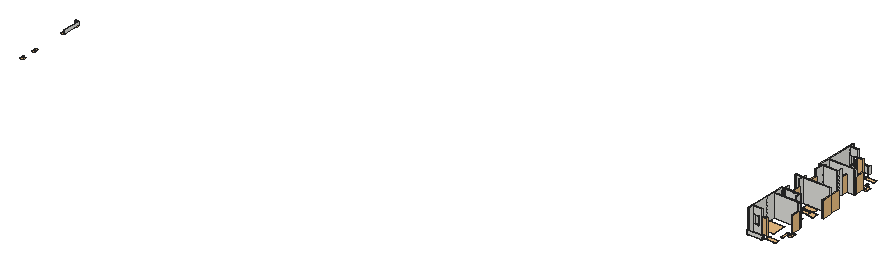
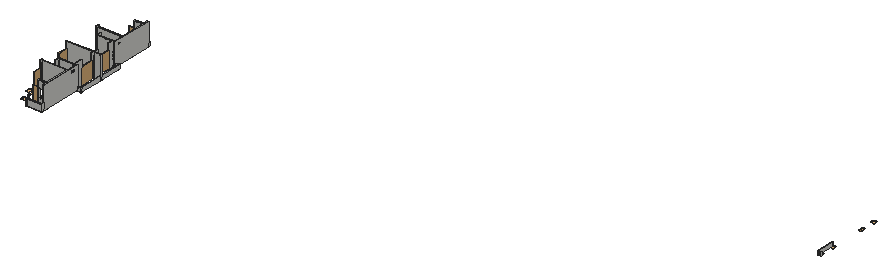
# SketchUp Ruby script. Lengths in inches.
U = 1.inch
M = Sketchup.active_model
def pt(a) = Geom::Point3d.new(a.map { |v| v * U })
def face(e, loops, mat)
  f = e.add_face(loops[0].map { |a| pt(a) })
  loops[1..].each { |l| e.add_face(l.map { |a| pt(a) }).erase! }
  f.material = f.back_material = mat if mat
  f
end
# faces: each face lists its corners as indices into pts; further lists are holes
def faces(e, pts, list, mat = nil) = list.each { |f| face(e, (f[0].is_a?(Array) ? f : [f]).map { |l| l.map { |i| pts[i] } }, mat) }
# xy, xz, yz: faces in a plane at the given z, y or x. An outline is a flat list of corners, or four numbers for a rectangle; further outlines are holes
def ring(l) = l.size == 4 ? [[l[0], l[1]], [l[2], l[1]], [l[2], l[3]], [l[0], l[3]]] : l.each_slice(2).to_a
def flat(e, list, mat, &to3) = list.each { |f| face(e, (f[0].is_a?(Array) ? f : [f]).map { |l| ring(l).map { |u, v| to3.(u, v) } }, mat) }
def xy(e, z, list, mat = nil) = flat(e, list, mat) { |x, y| [x, y, z] }
def xz(e, y, list, mat = nil) = flat(e, list, mat) { |x, z| [x, y, z] }
def yz(e, x, list, mat = nil) = flat(e, list, mat) { |y, z| [x, y, z] }
def lines(e, pts, list) = list.each { |a, b| e.add_line(pt(pts[a]), pt(pts[b])) }
# prism: a flat outline (further loops are holes) pulled along v
def prism(e, loops, v, mat = nil)
  f = face(e, loops, mat); d = Geom::Vector3d.new(v.map { |x| x * U })
  f.pushpull(f.normal.samedirection?(d) ? d.length : -d.length)
end
def box(e, o, s, mat = nil) = prism(e, [[o, [o[0] + s[0], o[1], o[2]], [o[0] + s[0], o[1] + s[1], o[2]], [o[0], o[1] + s[1], o[2]]]], [0, 0, s[2]], mat)
def at(x, y, z, deg = 0) = Geom::Transformation.translation(pt([x, y, z])) * Geom::Transformation.rotation(ORIGIN, Z_AXIS, deg.degrees)
def axes(o, x, y, z) = Geom::Transformation.new([*x, 0, *y, 0, *z, 0, *pt(o).to_a, 1])
def part(name) = M.definitions.add(name)
# library, detail: a bought-in or finely detailed component or shape, given as its bounding box
def library(name, o, s) = part(name).tap { |d| box(d.entities, o, s) }
def detail(e, o, s) = box(e.add_group.entities, o, s)
def put(e, d, t, mat = nil) = e.add_instance(d, t).tap { |i| i.material = mat if mat }
def group(e, t, mat = nil) = e.add_group.tap { |g| g.transformation = t; g.material = mat if mat }.entities
root = M.entities
M.materials.add("M09_Shadow_Night").color = [0, 0, 0]
c1 = library("TREE-26",[-60.96,-72.91,0],[121.92,134.74,0.01])
c2 = part("Group\#14")
xy(c2.entities,0,[[0,0,4.05,3.45],[0,3.45,4.05,88.84],[-13.95,88.84,0,93],[0,88.84,4.05,93]])
xy(c2.entities,18,[[0,0,4.05,88.84],[-13.95,88.84,0,93],[0,88.84,4.05,93]],"M09_Shadow_Night")
xz(c2.entities,0,[[0,0,4.05,18]])
xz(c2.entities,88.84,[[-13.95,0,0,18]])
xz(c2.entities,93,[[-13.95,0,4.05,18]])
yz(c2.entities,-13.95,[[88.84,0,93,18]])
yz(c2.entities,0,[[0,0,3.45,18],[3.45,0,88.84,18]])
yz(c2.entities,4.05,[[0,0,93,18]])
c3 = library("porta correr aluminio",[0,0,0],[4.49,110.28,83.35])
c4 = library("ghgjg",[-265.23,-341.01,0],[530.46,682.02,0.01])
c5 = library("VVVV",[-3.39,-3.68,0],[6.78,7.36,0.01])
c6 = part("Group\#13")
xy(c6.entities,0,[[0,0,4,3.01],[80,0,84,8],[0,3.01,4,8],[0,8,4,12],[4,8,80,12],
  [80,8,84,12]])
xy(c6.entities,36,[[0,0,4,12],[80,0,84,12],[4,8,80,12]],"M09_Shadow_Night")
xz(c6.entities,0,[[0,0,4,36],[80,0,84,36]])
xz(c6.entities,8,[[4,0,80,36]])
xz(c6.entities,12,[[0,0,80,36],[80,0,84,36]])
yz(c6.entities,0,[[0,0,12,36]])
yz(c6.entities,4,[[0,0,3.01,36],[3.01,0,8,36]])
yz(c6.entities,80,[[0,0,8,36],[8,0,12,36]])
yz(c6.entities,84,[[0,0,12,36]])
c7 = part("Group\#6")
xy(c7.entities,0,[[0,-8,80,-4],[80,-8,84,-4],[0,-4,4,0],[80,-4,84,4],[0,0,4,4]])
xy(c7.entities,20,[[0,-8,84,-8,84,4,80,4,80,-4,4,-4,4,4,0,4]],"M09_Shadow_Night")
xz(c7.entities,-8,[[0,0,84,20]])
xz(c7.entities,-4,[[4,0,80,20]])
xz(c7.entities,4,[[0,0,4,20],[80,0,84,20]])
yz(c7.entities,0,[[-8,0,4,20]])
yz(c7.entities,4,[[-4,0,0,20],[0,0,4,20]])
yz(c7.entities,80,[[-4,0,4,20]])
yz(c7.entities,84,[[-8,0,-4,20],[-4,0,4,20]])
c8 = library("double bed",[-999.9375,-1062.5,0],[1999.875,2125,0.01])
c9 = part("tgr")
p = [[-2.37,-3.35,0],[-2.37,-2.82,0],[-2.73,-2.82,0],[-2.73,-2.68,0],[-3.71,-2.68,0],[-3.71,-3.35,0],
  [-2.37,3.35,0],[-2.37,2.82,0],[-2.73,2.82,0],[-2.73,2.68,0],[-3.71,2.68,0],[-3.71,3.35,0],
  [3.71,-2.82,0],[-2.37,-2.46,0],[3.71,-2.46,0],[3.7,-2.46,0],[3.63,-2.07,0],[3.53,-1.68,0],
  [3.41,-1.3,0],[3.27,-0.93,0],[3.1,-0.57,0],[2.91,-0.22,0],[2.7,0.12,0],[2.46,0.4375,0],
  [2.21,0.74,0],[1.93,1.03,0],[1.64,1.3,0],[1.33,1.55,0],[1.01,1.79,0],[0.67,1.99,0],
  [0.32,2.18,0],[-0.04,2.35,0],[-0.41,2.49,0],[-0.8,2.6,0],[-1.18,2.69,0],[-1.58,2.76,0],
  [-1.97,2.8,0]]
lines(c9.entities,p,[[0,1],[1,2],[2,3],[3,4],[4,5],[5,0],[6,7],[7,8],[8,9],[9,10],[10,11],[11,6],
  [1,12],[13,14],[1,13],[12,14],[15,16],[16,17],[17,18],[18,19],[19,20],[20,21],[21,22],[22,23],
  [23,24],[24,25],[25,26],[26,27],[27,28],[28,29],[29,30],[30,31],[31,32],[32,33],[33,34],[34,35],
  [35,36],[36,7]])
c10 = library("Group\#51",[0,0,0],[6.9375,42,86.5])
c11 = library("HYHHYHYHYHYHY",[-2.09,-4.54,0],[4.18,9.08,0.01])
c12 = library("BFGFV",[-4.32,-2.51,0],[8.64,5.02,0.01])
c13 = library("lcd-01",[-577.99,-134.75,0],[1155.98,269.5,0.01])
c14 = library("JEEW",[-211.14,-299.86,0],[422.28,599.72,0.01])
c15 = library("Group\#49",[0,0,0],[8.31,30,84])
c16 = library("Component\#1",[961.32,38.58,0],[54,24,0.01])
c17 = library("Component\#3",[961.32,686.58,0],[54,18,0.01])
c18 = part("EGWF")
p = [[2.59,-3.49,0],[2.59,-3.09,0],[2.85,-3.09,0],[2.85,-2.99,0],[3.58,-2.99,0],[3.58,-3.49,0],
  [2.59,3.49,0],[2.59,3.09,0],[2.85,3.09,0],[2.85,2.99,0],[3.58,2.99,0],[3.58,3.49,0],
  [-3.58,-3.09,0],[2.59,-2.82,0],[-3.58,-2.82,0],[2.2,3.07,0],[1.81,3.04,0],[1.42,2.97,0],
  [1.03,2.89,0],[0.66,2.78,0],[0.29,2.64,0],[-0.07,2.48,0],[-0.42,2.3,0],[-0.76,2.1,0],
  [-1.08,1.875,0],[-1.39,1.63,0],[-1.68,1.37,0],[-1.96,1.09,0],[-2.21,0.79,0],[-2.45,0.48,0],
  [-2.67,0.15,0],[-2.86,-0.1875,0],[-3.04,-0.54,0],[-3.1875,-0.9,0],[-3.32,-1.28,0],[-3.42,-1.66,0],
  [-3.5,-2.04,0],[-3.55,-2.43,0]]
lines(c18.entities,p,[[0,1],[1,2],[2,3],[3,4],[4,5],[5,0],[6,7],[7,8],[8,9],[9,10],[10,11],[11,6],
  [1,12],[13,14],[1,13],[12,14],[7,15],[15,16],[16,17],[17,18],[18,19],[19,20],[20,21],[21,22],
  [22,23],[23,24],[24,25],[25,26],[26,27],[27,28],[28,29],[29,30],[30,31],[31,32],[32,33],[33,34],
  [34,35],[35,36],[36,37],[37,14]])
c19 = part("feeeeeeeeee")
p = [[-2.68,3.51,0],[-2.68,3.16,0],[-2.92,3.16,0],[-2.92,3.07,0],[-3.56,3.07,0],[-3.56,3.51,0],
  [-2.68,-3.51,0],[-2.68,-3.16,0],[-2.92,-3.16,0],[-2.92,-3.07,0],[-3.56,-3.07,0],[-3.56,-3.51,0],
  [3.56,3.16,0],[-2.68,2.93,0],[3.56,2.93,0],[-2.48,-3.13,0],[-2.04,-3.07,0],[-1.61,-2.98,0],
  [-1.1875,-2.86,0],[-0.77,-2.72,0],[-0.36,-2.55,0],[0.03,-2.35,0],[0.41,-2.13,0],[0.78,-1.88,0],
  [1.125,-1.62,0],[1.46,-1.32,0],[1.77,-1.01,0],[2.06,-0.68,0],[2.33,-0.33,0],[2.57,0.03,0],
  [2.79,0.42,0],[2.99,0.81,0],[3.16,1.22,0],[3.3,1.63,0],[3.41,2.06,0],[3.5,2.49,0]]
lines(c19.entities,p,[[0,1],[1,2],[2,3],[3,4],[4,5],[5,0],[6,7],[7,8],[8,9],[9,10],[10,11],[11,6],
  [1,12],[13,14],[1,13],[12,14],[8,15],[15,16],[16,17],[17,18],[18,19],[19,20],[20,21],[21,22],
  [22,23],[23,24],[24,25],[25,26],[26,27],[27,28],[28,29],[29,30],[30,31],[31,32],[32,33],[33,34],
  [34,35],[35,14]])
xy(root,246,[[3708.46,942.875,3762.46,966.875]])
put(root,c1,axes([371.8,298.64,246],[0,0.1317,0],[0.1317,0,0],[0,0,0.1317]))
put(root,c1,axes([371.8,222.26,246],[0,0.1317,0],[0.1317,0,0],[0,0,0.1317]))
put(root,c1,axes([371.8,567.61,246],[0,0.1317,0],[0.1317,0,0],[0,0,0.1317]))
put(root,c1,axes([371.8,491.09,246],[0,0.1317,0],[0.1317,0,0],[0,0,0.1317]))
put(root,c2,at(376.15,484.34,246))
put(root,c1,axes([3611.24,1266.81,246],[0,0.1317,0],[0.1317,0,0],[0,0,0.1317]))
put(root,c1,axes([3611.24,1401.53,246],[0,0.1317,0],[0.1317,0,0],[0,0,0.1317]))
put(root,c1,axes([3611.24,1285.67,246],[0,0.1317,0],[0.1317,0,0],[0,0,0.1317]))
put(root,c1,axes([3611.24,1162.38,246],[0,0.1317,0],[0.1317,0,0],[0,0,0.1317]))
put(root,c1,axes([3635.38,935.84,246],[0,0.1317,0],[0.1317,0,0],[0,0,0.1317]))
put(root,c1,axes([3637.36,1629.4,246],[0,0.1317,0],[0.1317,0,0],[0,0,0.1317]))
put(root,c3,axes([3644.59,1182.875,246.65],[-1.89519,0,0],[0,0.65291,0],[0,0,1]))
put(root,c3,axes([3644.59,1292.48,246.65],[-1.89519,0,0],[0,0.65291,0],[0,0,1]))
put(root,c4,axes([3644.1,1128.875,246],[0,-0.04,0],[-0.04,0,0],[0,0,0.04]))
put(root,c4,axes([3644.1,1434.875,246],[0,-0.04,0],[-0.04,0,0],[0,0,0.04]))
put(root,c5,axes([3663.08,1221.31,246],[4.47564,0,0],[0,-4.47564,0],[0,0,4.47564]))
put(root,c5,axes([3663.08,1330.86,246],[4.47564,0,0],[0,4.47564,0],[0,0,4.47564]))
put(root,c6,at(3624.46,1626.8,246))
put(root,c7,at(3624.46,932.875,246))
put(root,c8,axes([3669.72,1035.82,246],[0,-0.03695,0],[-0.03695,0,0],[0,0,0.03695]))
put(root,c8,axes([3669.72,1520.61,246],[0,-0.03695,0],[-0.03695,0,0],[0,0,0.03695]))
put(root,c9,axes([3687.46,1613.47,246],[0,4.47464,0],[-4.47464,0,0],[0,0,4.47464]))
put(root,c10,axes([3702.46,1595.22,246],[0,0.85622,0],[-0.71429,0,0],[0,0,0.97071]))
put(root,c9,axes([3687.46,950.27,246],[0,-4.47464,0],[-4.47464,0,0],[0,0,4.47464]))
put(root,c10,axes([3674.86,968.53,246],[0,-0.85622,0],[0.65714,0,0],[0,0,0.9711]))
g1 = group(root,at(3624.46,1619.08,246))
xy(g1,0,[[12,-255.51,18,-214.2],[0,-214.2,6,-208.2],[6,-214.2,12,-208.2],[12,-214.2,18,-208.2],[18,-214.2,94,-208.2],
  [94,-214.2,100,-208.2],[0,-208.2,6,-160.2],[94,-208.2,100,-190.2],[0,-160.2,6,-154.2],[6,-160.2,138,-154.2],
  [138,-160.2,144,-154.2],[0,-154.2,6,-116.77],[138,-154.2,144,-148.2],[0,-116.77,6,-80.17],[0,-80.17,6,-22.2],
  [0,-22.2,6,-16.2],[6,-22.2,48,-16.2],[0,-16.2,6,0],[0,0,6,7.73]])
xy(g1,36,[[8,-22.2,46,-16.2]])
xy(g1,84,[[8,-22.2,46,-16.2]])
xy(g1,96,[[0,-196.2,6,-172.2]])
xy(g1,108,[[0,-196.2,6,-172.2]])
xy(g1,120,[[12,-255.51,18,-214.2],[0,-214.2,6,-208.2],[6,-214.2,12,-208.2],[12,-214.2,18,-208.2],[18,-214.2,94,-208.2],
  [94,-214.2,100,-208.2],[0,-208.2,6,-160.2],[94,-208.2,100,-190.2],[0,-160.2,6,-154.2],[6,-160.2,138,-154.2],
  [138,-160.2,144,-154.2],[0,-154.2,6,-22.2],[138,-154.2,144,-148.2],[0,-22.2,6,-16.2],[6,-22.2,48,-16.2],
  [0,-16.2,6,0],[0,0,6,7.73]])
xz(g1,-255.51,[[12,0,18,120]])
xz(g1,-214.2,[[0,0,6,120],[6,0,12,120],[12,0,18,120],[18,0,94,120],[94,0,100,120]])
xz(g1,-208.2,[[6,0,12,120],[12,0,18,120],[18,0,94,120],[94,0,100,120]])
xz(g1,-196.2,[[0,96,6,108]])
xz(g1,-190.2,[[94,0,100,120]])
xz(g1,-172.2,[[0,96,6,108]])
xz(g1,-160.2,[[6,0,138,120],[138,0,144,120]])
xz(g1,-154.2,[[6,0,138,120],[138,0,144,120]])
xz(g1,-148.2,[[138,0,144,120]])
xz(g1,-22.2,[[[6,0,48,120],[8,36,46,84]]])
xz(g1,-16.2,[[[6,0,48,120],[8,36,46,84]]])
xz(g1,7.73,[[0,0,6,120]])
yz(g1,0,[[[-214.2,0,7.73,120],[-196.2,96,-172.2,108]]])
yz(g1,6,[[-214.2,0,-208.2,120],[[-208.2,0,-160.2,120],[-196.2,96,-172.2,108]],[-160.2,0,-154.2,120],[-154.2,0,-22.2,120],[-22.2,0,-16.2,120],
  [-16.2,0,0,120],[0,0,7.73,120]])
yz(g1,8,[[-22.2,36,-16.2,84]])
yz(g1,12,[[-255.51,0,-214.2,120],[-214.2,0,-208.2,120]])
yz(g1,18,[[-255.51,0,-214.2,120],[-214.2,0,-208.2,120]])
yz(g1,46,[[-22.2,36,-16.2,84]])
yz(g1,48,[[-22.2,0,-16.2,120]])
yz(g1,94,[[-214.2,0,-208.2,120],[-208.2,0,-190.2,120]])
yz(g1,100,[[-214.2,0,-208.2,120],[-208.2,0,-190.2,120]])
yz(g1,138,[[-160.2,0,-154.2,120],[-154.2,0,-148.2,120]])
yz(g1,144,[[-160.2,0,-154.2,120],[-154.2,0,-148.2,120]])
g2 = group(g1,at(-2.625,-212.2,0))
xy(g2,0,[[2.625,-470,8.625,-446],[2.625,-446,8.625,-440],[8.625,-446,53.03,-440],[2.625,-440,8.625,-352.75],[2.625,-352.75,8.625,-308],
  [140.625,-317.47,146.625,-308],[2.625,-308,8.625,-302],[8.625,-308,140.625,-302],[140.625,-308,146.625,-302],[2.625,-302,8.625,-254],
  [96.625,-272,102.625,-254],[-21.375,-254,-17.27,-250],[-17.27,-254,2.625,-250],[2.625,-254,8.625,-250],[8.625,-254,14.625,-250],
  [14.625,-254,20.625,-250],[20.625,-254,96.625,-250],[96.625,-254,102.625,-250],[-21.375,-250,-17.27,-133.43],[2.625,-250,8.625,-248],
  [8.625,-250,14.625,-248],[14.625,-250,20.625,-248],[20.625,-250,96.625,-248],[96.625,-250,102.625,-248],[14.625,-248,20.625,-224],
  [14.625,-152,20.625,-133.43],[-21.375,-133.43,-17.27,-127.79],[-17.27,-133.43,14.625,-127.79],[14.625,-133.43,20.625,-127.79],[20.625,-133.43,164.625,-127.79],
  [-21.375,-127.79,-17.27,0],[14.625,-127.79,20.625,-114.45],[-21.375,0,-17.27,4],[-17.27,0,2.625,4]])
xy(g2,20,[[-21.375,-254,2.625,-250],[-21.375,-250,-17.27,-133.43],[-21.375,-127.79,-17.27,0],[-21.375,0,2.625,4]],"M09_Shadow_Night")
xy(g2,36,[[11.33,-446,41.03,-440]])
xy(g2,84,[[11.33,-446,41.03,-440]])
xy(g2,96,[[2.625,-290,8.625,-266]])
xy(g2,108,[[2.625,-290,8.625,-266]])
xy(g2,119.9375,[[96.625,-272,102.625,-254]])
xy(g2,120,[[2.625,-470,8.625,-446],[2.625,-446,8.625,-440],[8.625,-446,53.03,-440],[2.625,-440,8.625,-352.75],[2.625,-352.75,8.625,-308],
  [140.625,-317.47,146.625,-308],[2.625,-308,8.625,-302],[8.625,-308,140.625,-302],[140.625,-308,146.625,-302],[2.625,-302,8.625,-254],
  [2.625,-254,8.625,-248],[8.625,-254,14.625,-248],[14.625,-254,20.625,-248],[20.625,-254,96.625,-248],[96.625,-254,102.625,-248],
  [14.625,-248,20.625,-224],[14.625,-152,20.625,-133.43],[-21.375,-133.43,-17.27,-127.79],[-17.27,-133.43,14.625,-127.79],[14.625,-133.43,20.625,-127.79],
  [20.625,-133.43,164.625,-127.79],[14.625,-127.79,20.625,-114.45]])
xz(g2,-470,[[2.625,0,8.625,120]])
xz(g2,-446,[[[8.625,0,53.03,120],[11.33,36,41.03,84]]])
xz(g2,-440,[[[8.625,0,53.03,120],[11.33,36,41.03,84]]])
xz(g2,-317.47,[[140.625,0,146.625,120]])
xz(g2,-308,[[8.625,0,140.625,120],[140.625,0,146.625,120]])
xz(g2,-302,[[8.625,0,140.625,120],[140.625,0,146.625,120]])
xz(g2,-290,[[2.625,96,8.625,108]])
xz(g2,-272,[[96.625,0,102.625,119.9375]])
xz(g2,-266,[[2.625,96,8.625,108]])
xz(g2,-254,[[-21.375,0,-17.27,20],[-17.27,0,2.625,20],[8.625,0,14.625,120],[14.625,0,20.625,120],[20.625,0,96.625,120],
  [96.625,0,102.625,119.9375],[96.625,119.9375,102.625,120]])
xz(g2,-250,[[-21.375,0,-17.27,20],[-17.27,0,2.625,20]])
xz(g2,-248,[[2.625,0,8.625,120],[8.625,0,14.625,120],[14.625,0,20.625,120],[20.625,0,96.625,120],[96.625,0,102.625,120]])
xz(g2,-224,[[14.625,0,20.625,120]])
xz(g2,-152,[[14.625,0,20.625,120]])
xz(g2,-133.43,[[-21.375,0,-17.27,20],[-17.27,0,14.625,120],[14.625,0,20.625,120],[20.625,0,164.625,120],[-21.375,20,-17.27,120]])
xz(g2,-127.79,[[-17.27,0,-17.27,20,-21.375,20,-21.375,120,14.625,120,14.625,0],[-21.375,0,-17.27,20],[14.625,0,20.625,120],[20.625,0,164.625,120]])
xz(g2,-114.45,[[14.625,0,20.625,120]])
xz(g2,0,[[-21.375,0,-17.27,20],[-17.27,0,2.625,20]])
xz(g2,4,[[-21.375,0,-17.27,20],[-17.27,0,2.625,20]])
yz(g2,-21.375,[[-254,0,-250,20],[-250,0,-133.43,20],[-133.43,0,-127.79,120],[-127.79,0,0,20],[0,0,4,20]])
yz(g2,-17.27,[[-250,0,-133.43,20],[-127.79,0,0,20]])
yz(g2,2.625,[[[-470,0,-470,120,-248,120,-248,0,-250,0,-250,20,-254,20,-254,0],[-290,96,-266,108]],[-254,0,-250,20],[0,0,4,20]])
yz(g2,8.625,[[-470,0,-446,120],[-446,0,-440,120],[-440,0,-352.75,120],[-352.75,0,-308,120],[-308,0,-302,120],
  [[-302,0,-254,120],[-290,96,-266,108]],[-254,0,-248,120]])
yz(g2,11.33,[[-446,36,-440,84]])
yz(g2,14.625,[[-254,0,-248,120],[-248,0,-224,120],[-152,0,-133.43,120],[-133.43,0,-127.79,120],[-127.79,0,-114.45,120]])
yz(g2,20.625,[[-254,0,-248,120],[-248,0,-224,120],[-152,0,-133.43,120],[-133.43,0,-127.79,120],[-127.79,0,-114.45,120]])
yz(g2,41.03,[[-446,36,-440,84]])
yz(g2,53.03,[[-446,0,-440,120]])
yz(g2,96.625,[[-272,0,-254,119.9375],[-254,0,-248,120]])
yz(g2,102.625,[[-272,0,-254,119.9375],[-254,0,-248,120]])
yz(g2,140.625,[[-317.47,0,-308,120],[-308,0,-302,120]])
yz(g2,146.625,[[-317.47,0,-308,120],[-308,0,-302,120]])
yz(g2,164.625,[[-133.43,0,-127.79,120]])
put(root,c11,axes([3697.74,1297.78,246],[0,-6.75189,0],[6.75189,0,0],[0,0,6.75189]))
put(root,c11,axes([3697.74,1254.4,246],[0,6.75189,0],[6.75189,0,0],[0,0,6.75189]))
put(root,c12,axes([3700.0625,1220.92,246],[4.3395,0,0],[0,-4.3395,0],[0,0,4.3395]))
put(root,c12,axes([3700.0625,1331.8,246],[4.3395,0,0],[0,4.3395,0],[0,0,4.3395]))
put(root,c13,axes([3701.34,1164.26,246],[0.04,0,0],[0,-0.04,0],[0,0,0.04]))
put(root,c13,axes([3701.34,1399.48,246],[0.04,0,0],[0,0.04,0],[0,0,0.04]))
put(root,c14,axes([3705.61,1143.83,246],[0,0.04284,0],[0.04284,0,0],[0,0,0.04284]))
put(root,c14,axes([3705.61,1419.92,246],[0,-0.04284,0],[-0.04284,0,0],[0,0,0.04284]))
put(root,c9,axes([3707.86,1119.875,246],[-4.47464,0,0],[0,4.47464,0],[0,0,4.47464]))
put(root,c9,axes([3707.86,1443.875,246],[-4.47464,0,0],[0,-4.47464,0],[0,0,4.47464]))
put(root,c10,axes([3726.12,1134.875,246],[-0.85622,0,0],[0,-0.71429,0],[0,0,0.9711]))
put(root,c15,at(3720.18,1428.875,246))
put(root,c16,at(2747.14,904.3,246))
put(root,c17,at(2747.14,904.3,246))
put(root,c5,axes([3736.66,1221.31,246],[-4.47564,0,0],[0,-4.47564,0],[0,0,4.47564]))
put(root,c5,axes([3736.66,1330.86,246],[-4.47564,0,0],[0,4.47564,0],[0,0,4.47564]))
put(root,c18,axes([3746.86,1491.875,246],[6.02515,0,0],[0,6.02515,0],[0,0,6.02515]))
put(root,c18,axes([3746.86,1071.875,246],[6.02515,0,0],[0,-6.02515,0],[0,0,6.02515]))
put(root,c13,axes([3757.07,1539.54,246],[0,-0.04,0],[0.04,0,0],[0,0,0.04]))
put(root,c13,axes([3757.07,1016.28,246],[0,-0.04,0],[0.04,0,0],[0,0,0.04]))
put(root,c19,axes([3762.12,1249.09,246],[-6.83664,0,0],[0,6.83664,0],[0,0,6.83664]))
put(root,c19,axes([3762.12,1303.09,246],[-6.83664,0,0],[0,-6.83664,0],[0,0,6.83664]))
put(root,c15,axes([3762.375,1050.875,246],[1,0,0],[0,1.28434,0],[0,0,1]))
put(root,c10,axes([3770.12,1512.875,246],[-0.85622,0,0],[0,-1,0],[0,0,0.9711]))
put(root,c14,axes([3777.5,1032.03,246],[-0.04284,0,0],[0,0.04284,0],[0,0,0.04284]))
put(root,c14,axes([3777.5,1531.72,246],[-0.04284,0,0],[0,0.04284,0],[0,0,0.04284]))
put(root,c10,axes([3788.12,1326.55,246],[-0.85622,0,0],[0,-1.13,0],[0,0,0.9711]))
put(root,c15,axes([3782.18,1225.09,246],[1,0,0],[0,1.6118,0],[0,0,1]))
